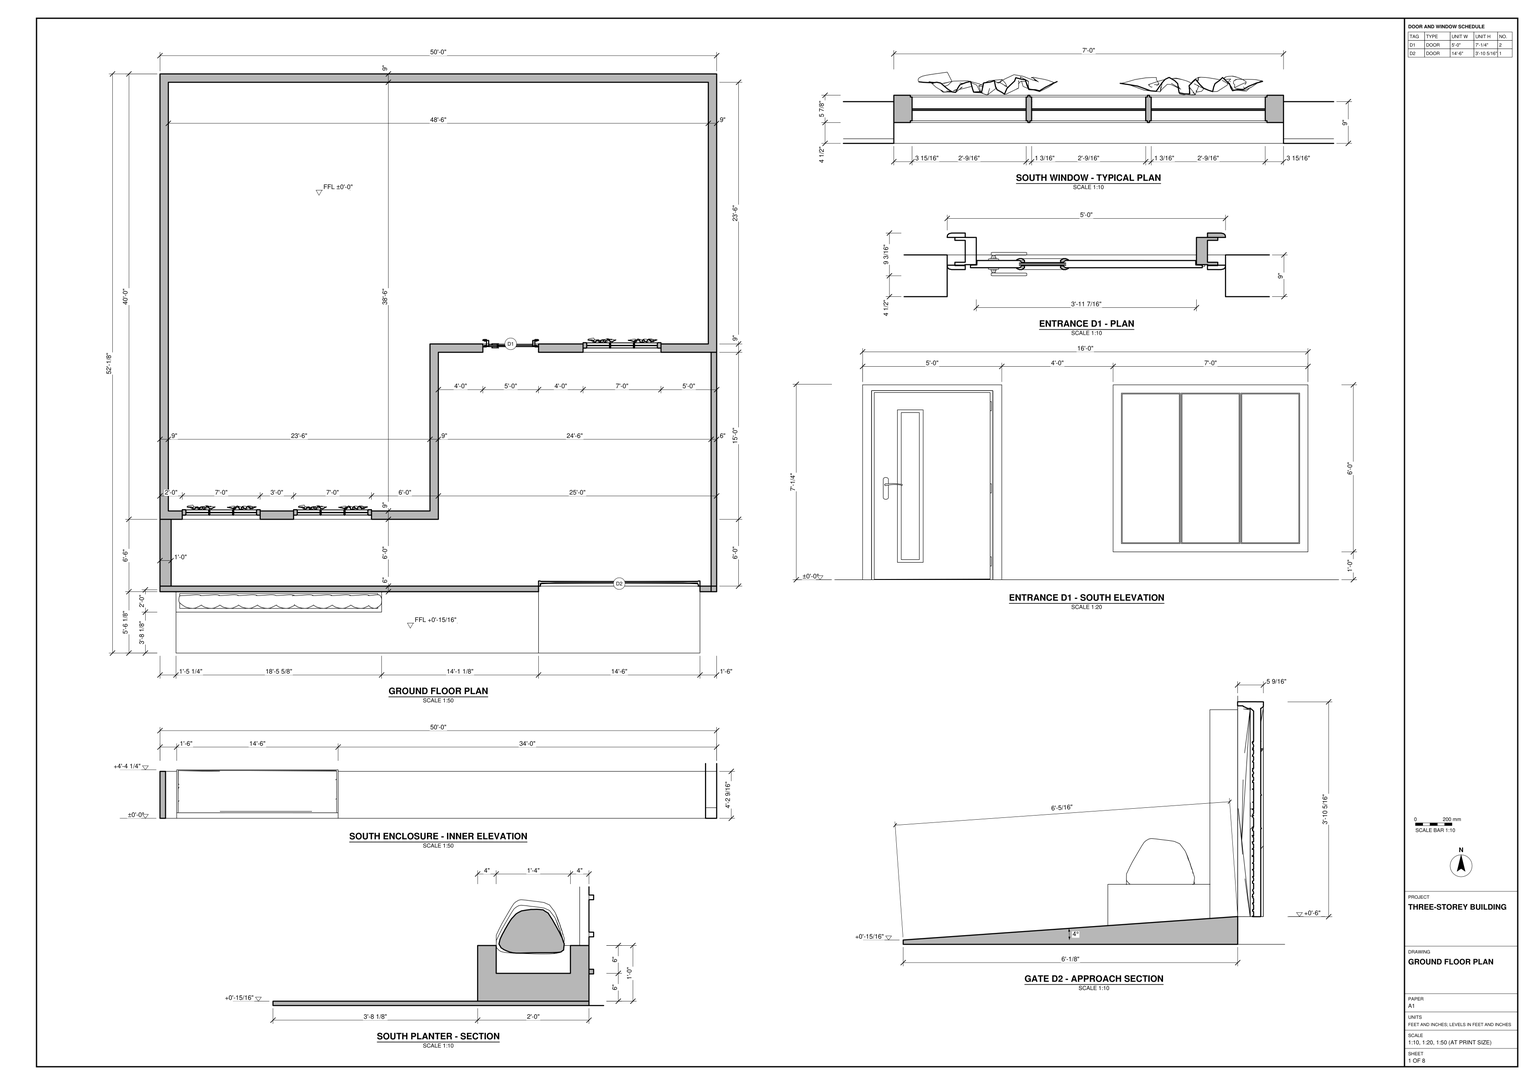
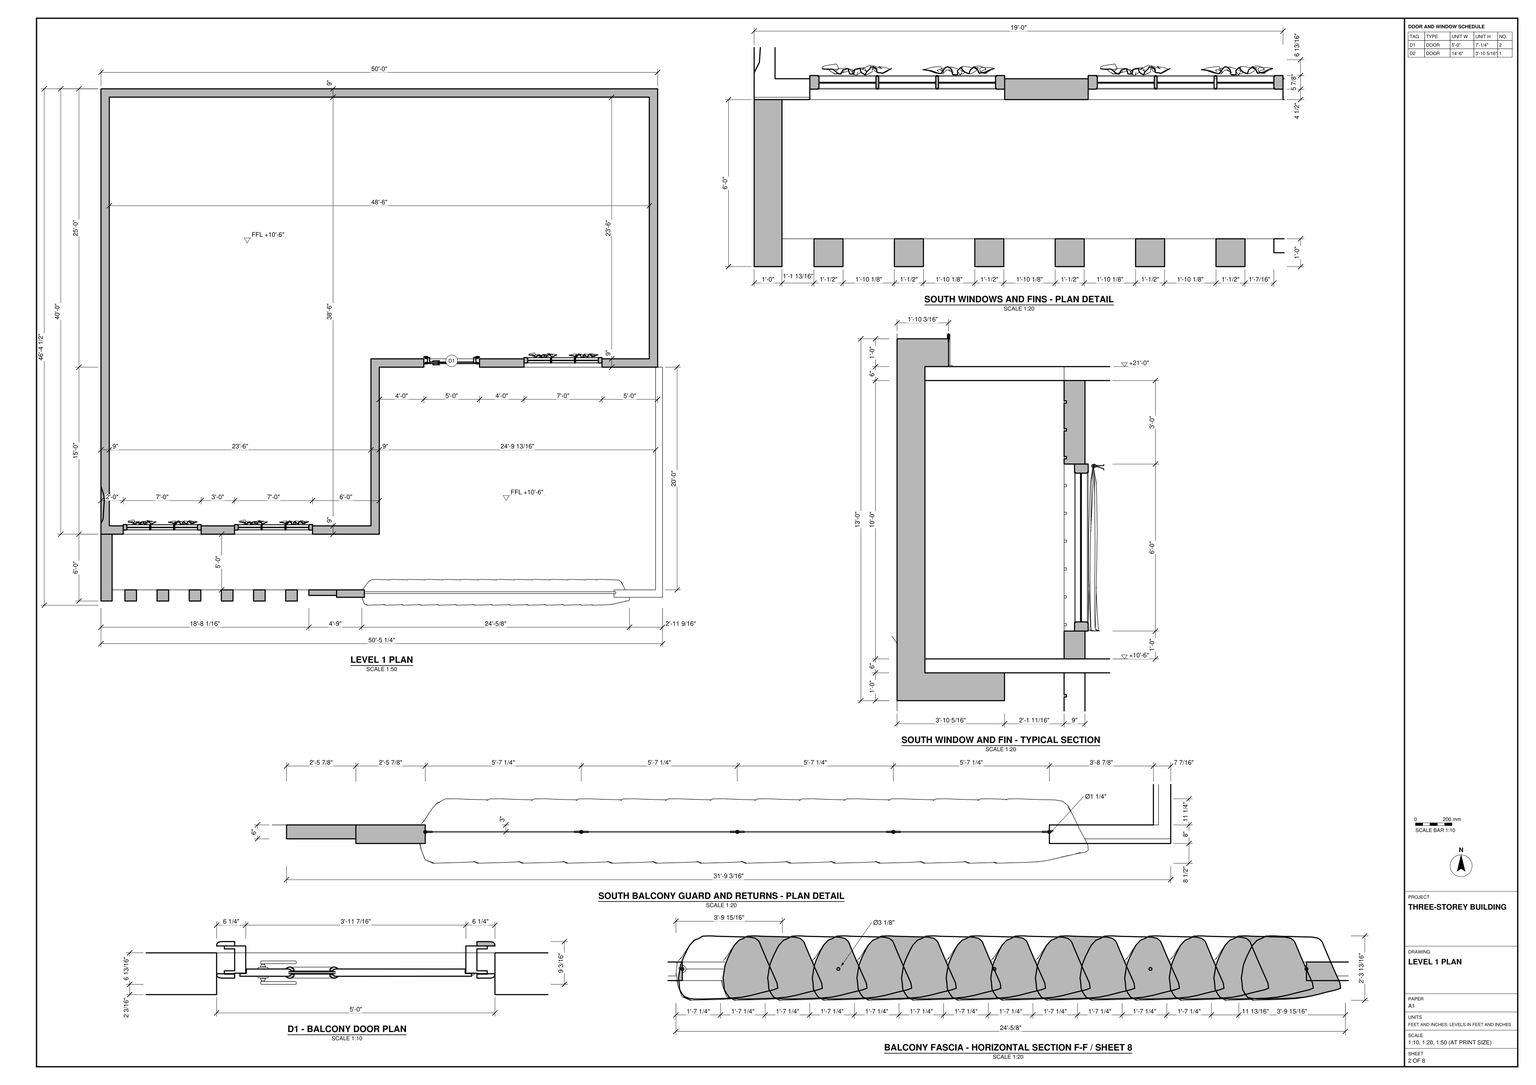
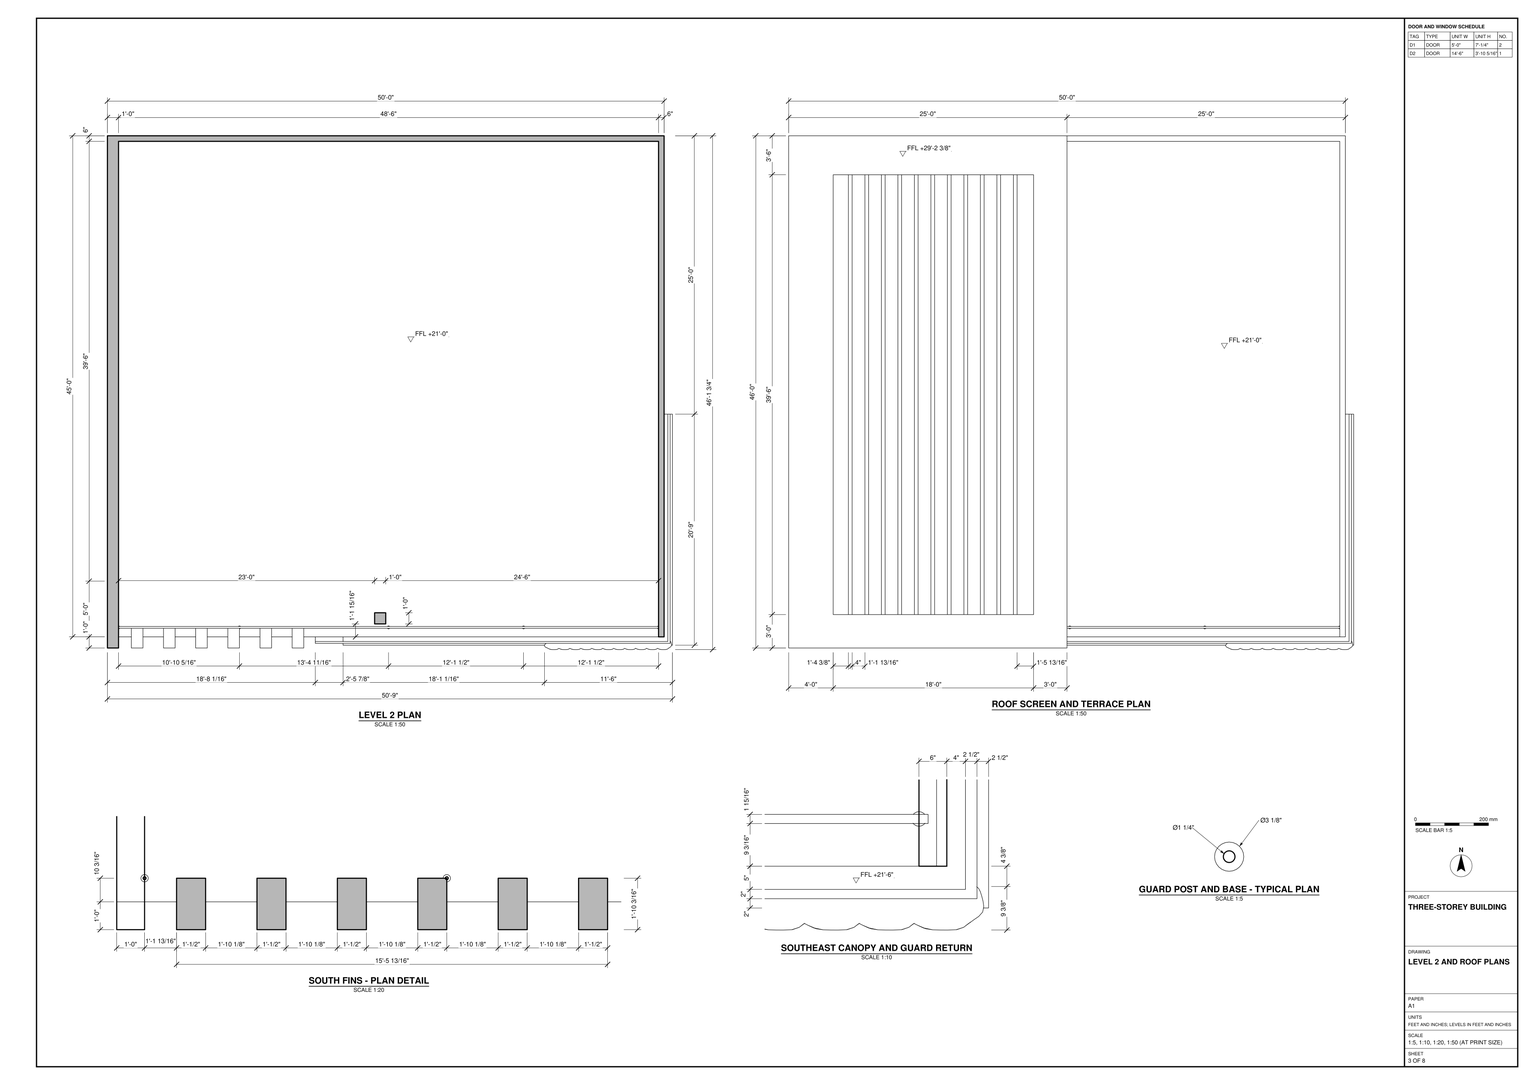
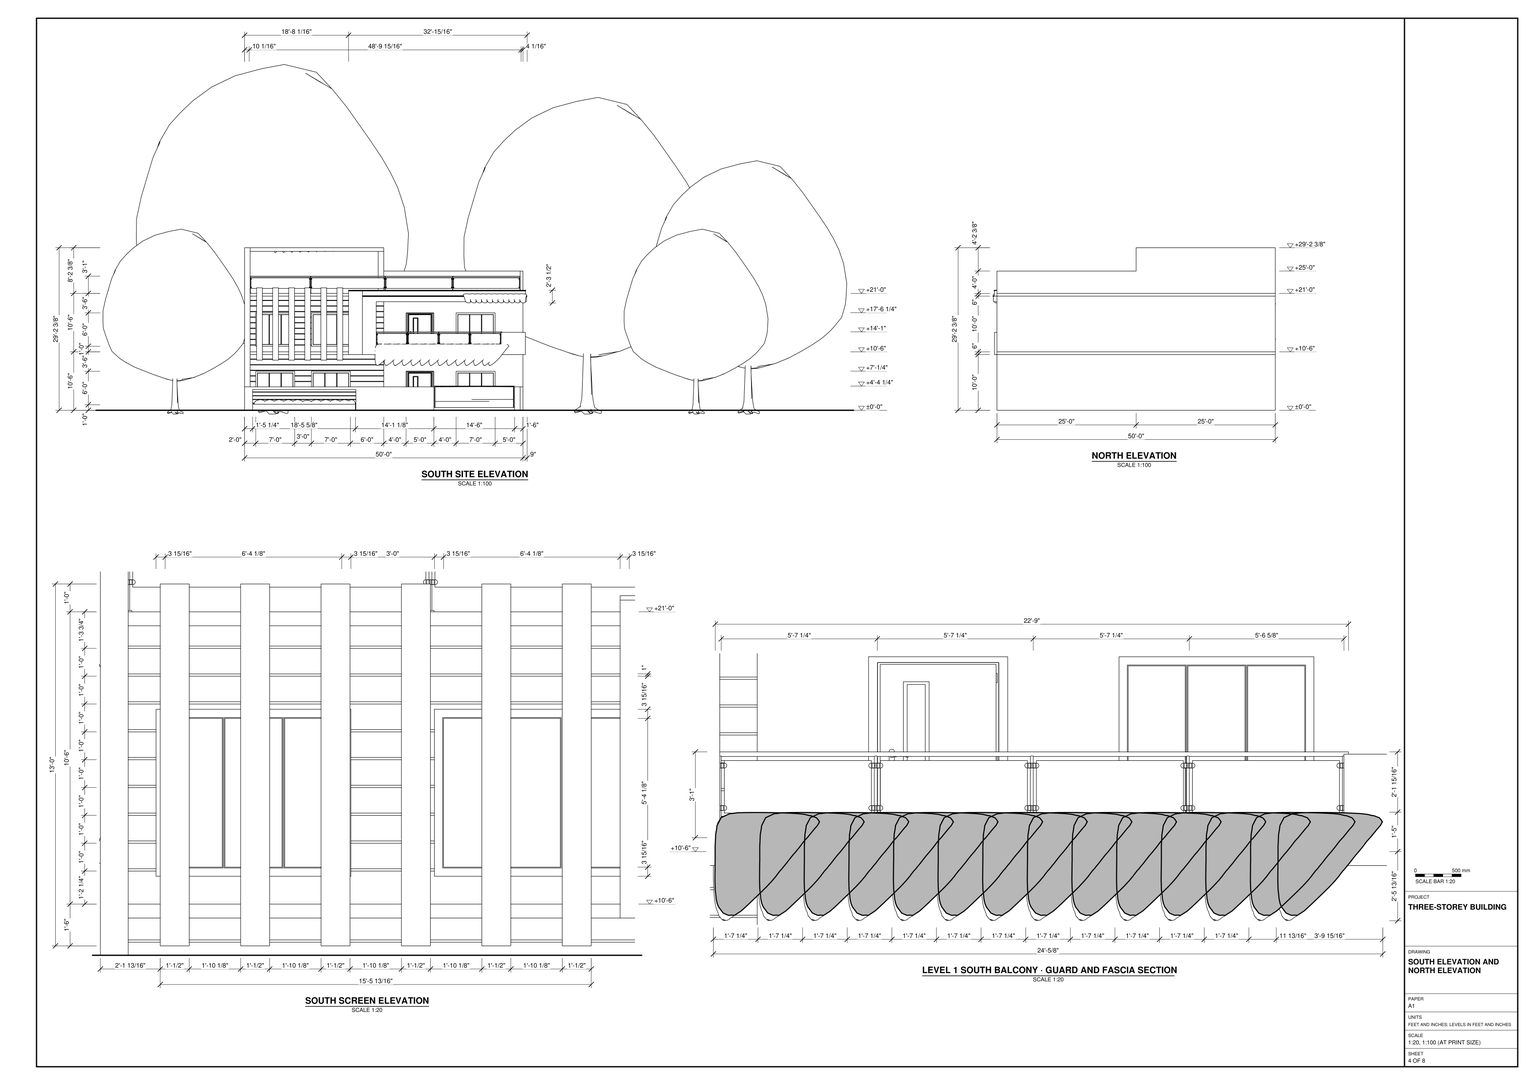
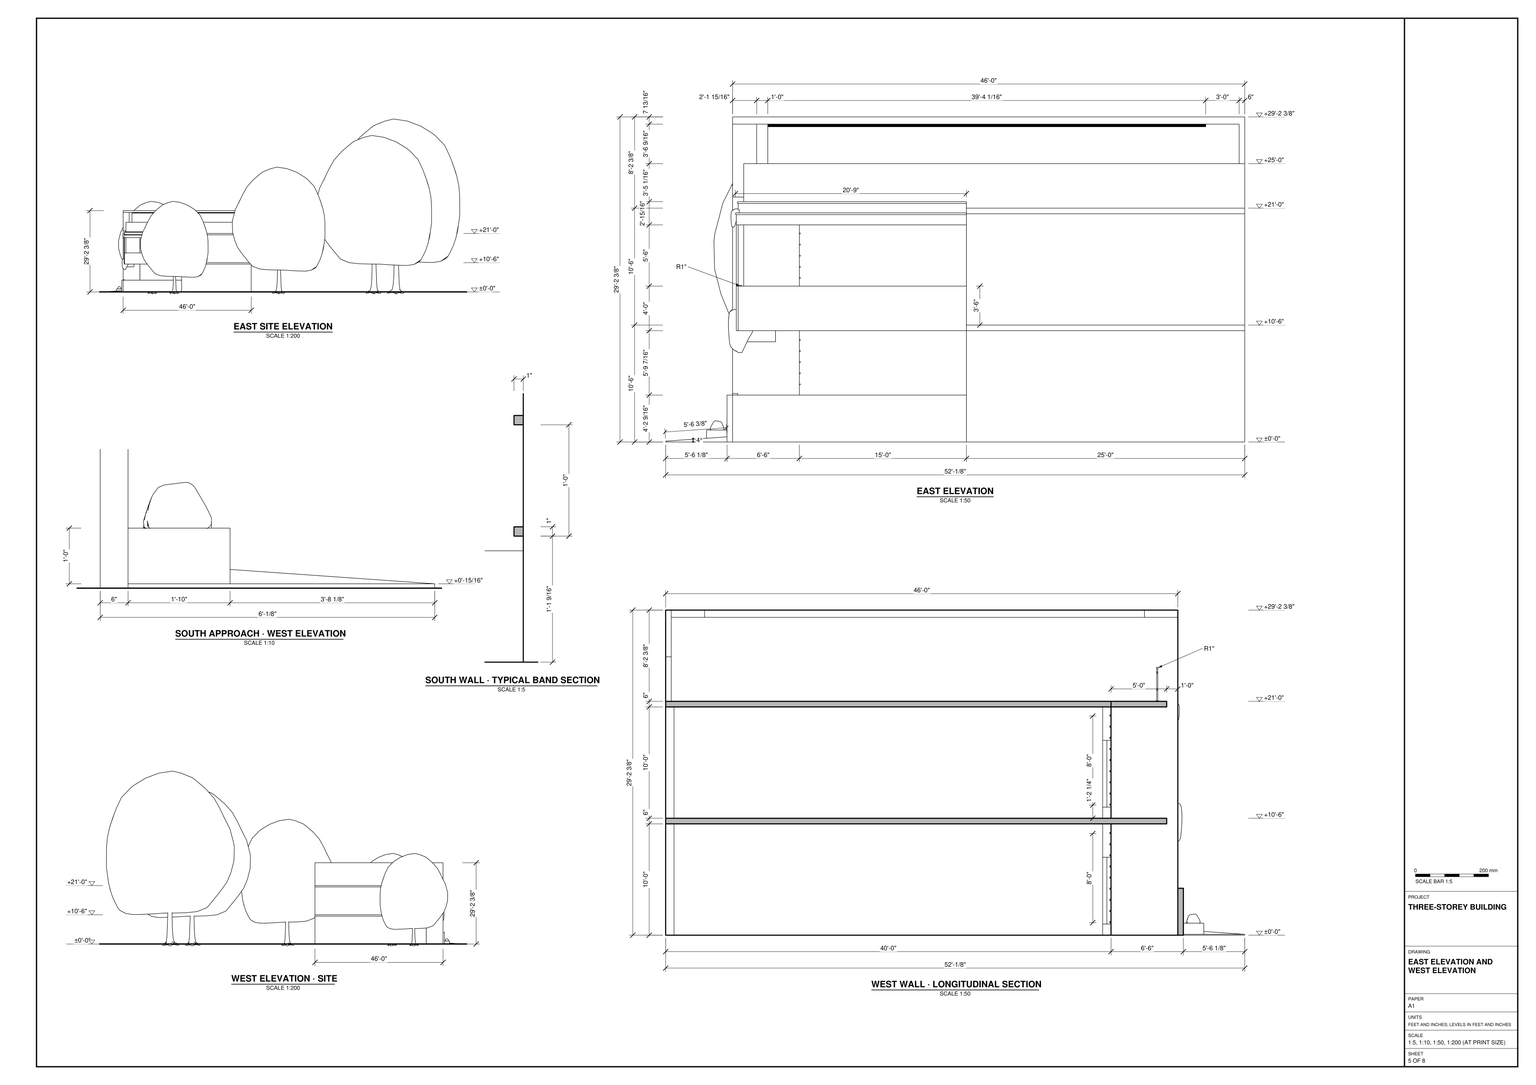
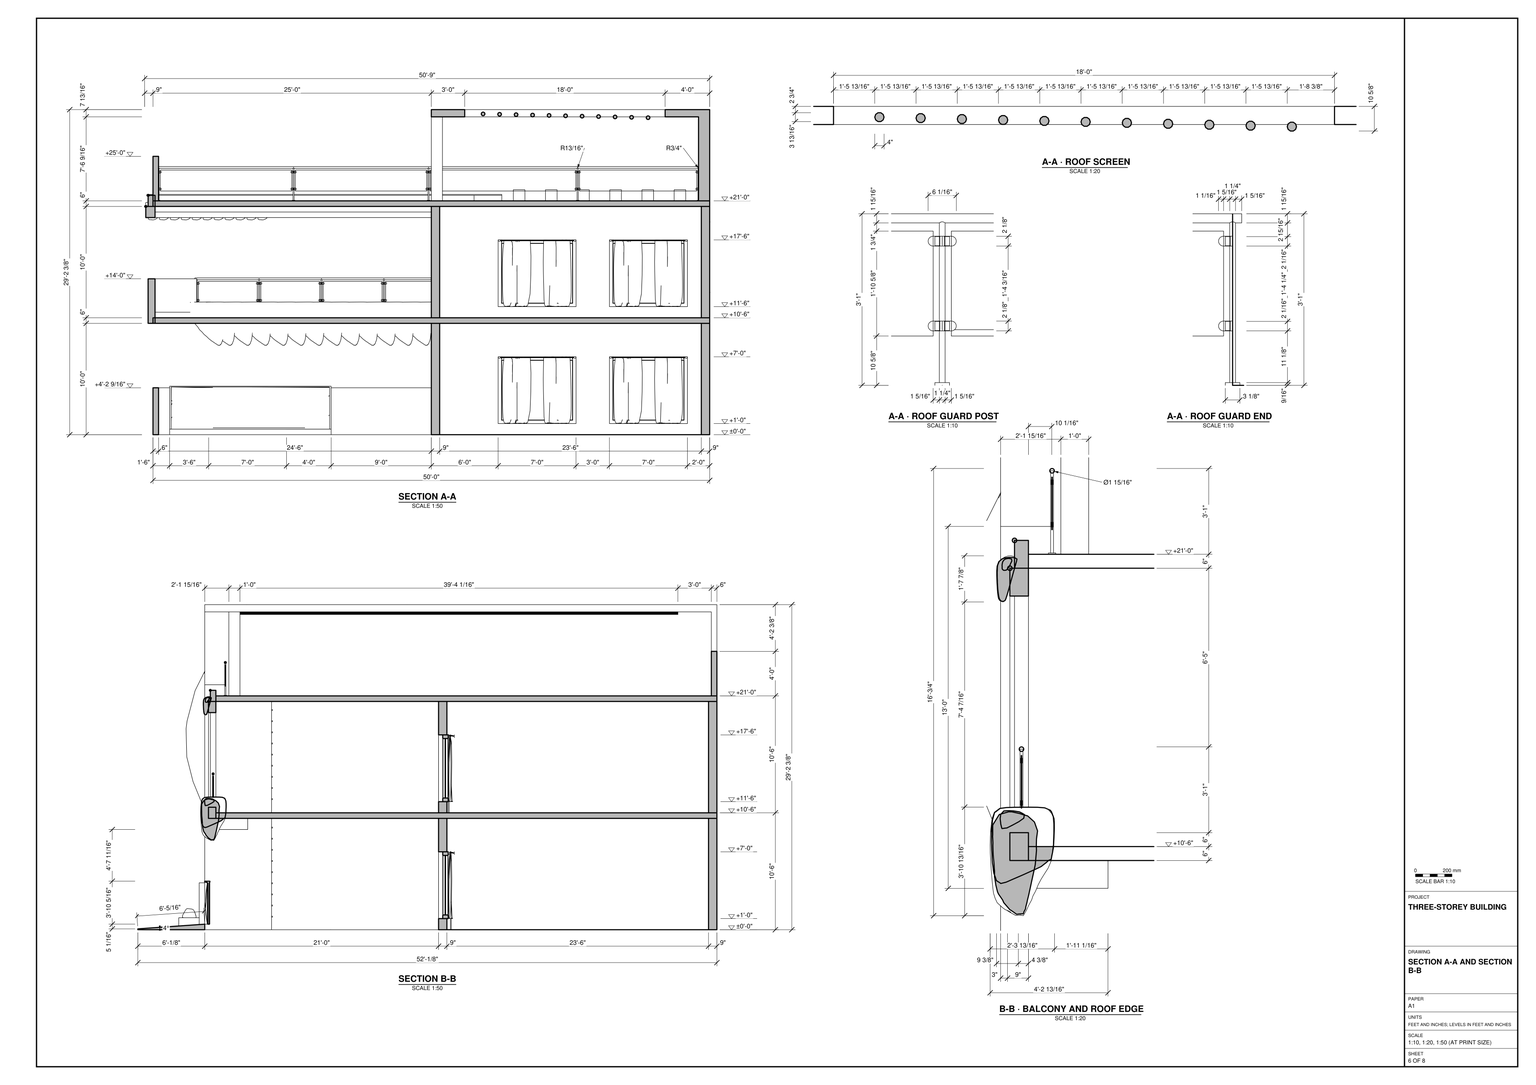
Build the three-storey building in SketchUp from task_files/diagram_01.pdf. Work in feet and inches. The complete model shall measure 133'-7 7/16" along X, 126'-11 1/8" along Y and 62'-9 9/16" along Z. These are the extents of the whole model, not the dimensions of the building footprint. Set the ground floor at ±0'-0", Level 1 at +10'-6" and Level 2 at +21'-0".

Use the floor plans to lay out the walls at their drawn thicknesses. On the two lower floors, the west wing projects south of the entrance wall. Fit the framed window units and doors into the wall openings. At ground level, model the south enclosure with the planter on the west and the sloping approach to the vehicle gate on the east.

Follow the sections for the floor slabs, projecting balcony edge and vertical fins in front of the Level 1 windows. Model the balcony's glass guard, its corner return and the repeating curved fascia. At roof level, distinguish the parallel strips of the roof screen on the west from the open terrace on the east. Decor and loose items, including planting and curtains, may be any suitable library components.

Keep shell elements such as walls, slabs and roof separate as groups or components. Keep each furniture or joinery piece shown separate, and use components for repeated parts. Save one SketchUp model as output_files/three_storey_building_south_balcony_and_roof_terrace.skp.

# SketchUp Ruby script. Lengths in inches.
U = 1.inch
M = Sketchup.active_model
def pt(a) = Geom::Point3d.new(a.map { |v| v * U })
def face(e, loops, mat)
  f = e.add_face(loops[0].map { |a| pt(a) })
  loops[1..].each { |l| e.add_face(l.map { |a| pt(a) }).erase! }
  f.material = f.back_material = mat if mat
  f
end
# faces: each face lists its corners as indices into pts; further lists are holes
def faces(e, pts, list, mat = nil) = list.each { |f| face(e, (f[0].is_a?(Array) ? f : [f]).map { |l| l.map { |i| pts[i] } }, mat) }
# xy, xz, yz: faces in a plane at the given z, y or x. An outline is a flat list of corners, or four numbers for a rectangle; further outlines are holes
def ring(l) = l.size == 4 ? [[l[0], l[1]], [l[2], l[1]], [l[2], l[3]], [l[0], l[3]]] : l.each_slice(2).to_a
def flat(e, list, mat, &to3) = list.each { |f| face(e, (f[0].is_a?(Array) ? f : [f]).map { |l| ring(l).map { |u, v| to3.(u, v) } }, mat) }
def xy(e, z, list, mat = nil) = flat(e, list, mat) { |x, y| [x, y, z] }
def xz(e, y, list, mat = nil) = flat(e, list, mat) { |x, z| [x, y, z] }
def yz(e, x, list, mat = nil) = flat(e, list, mat) { |y, z| [x, y, z] }
def lines(e, pts, list) = list.each { |a, b| e.add_line(pt(pts[a]), pt(pts[b])) }
# prism: a flat outline (further loops are holes) pulled along v
def prism(e, loops, v, mat = nil)
  f = face(e, loops, mat); d = Geom::Vector3d.new(v.map { |x| x * U })
  f.pushpull(f.normal.samedirection?(d) ? d.length : -d.length)
end
def box(e, o, s, mat = nil) = prism(e, [[o, [o[0] + s[0], o[1], o[2]], [o[0] + s[0], o[1] + s[1], o[2]], [o[0], o[1] + s[1], o[2]]]], [0, 0, s[2]], mat)
def at(x, y, z, deg = 0) = Geom::Transformation.translation(pt([x, y, z])) * Geom::Transformation.rotation(ORIGIN, Z_AXIS, deg.degrees)
def axes(o, x, y, z) = Geom::Transformation.new([*x, 0, *y, 0, *z, 0, *pt(o).to_a, 1])
def part(name) = M.definitions.add(name)
# library, detail: a bought-in or finely detailed component or shape, given as its bounding box
def library(name, o, s) = part(name).tap { |d| box(d.entities, o, s) }
def detail(e, o, s) = box(e.add_group.entities, o, s)
def put(e, d, t, mat = nil) = e.add_instance(d, t).tap { |i| i.material = mat if mat }
def group(e, t, mat = nil) = e.add_group.tap { |g| g.transformation = t; g.material = mat if mat }.entities
root = M.entities
M.materials.add("Marble White 604 35.18cm").color = [255, 255, 255]
M.materials.add("Metal for window").color = [30, 30, 30]
M.materials.add("Wall Paint Dusk Blue Matte 300cm").color = [122, 143, 157]
M.materials.add("Wall Paint Fine Grain 01 White 100cm").color = [188, 188, 188]
M.materials.add("Wall Paint Fine Grain 01 Yellow 100cm").color = [207, 190, 139]
c1 = library("Window with curtains",[-42,-36,-6.8],[84,72,12.68])
c2 = part("Component\#3")
prism(c2.entities,[[[0,-12,144],[0,10.1875,144],[0,10.1875,132],[0,0,132],[0,0,0],[0,34.3125,0],[0,34.3125,-12],[0,-12,-12]]],[12.51,0,0],"Wall Paint Dusk Blue Matte 300cm")
c3 = library("Door 29",[-21.26,-5.27,0],[42.52,9.21,84.25])
c4 = library("Lithodora diffusa 002",[-13.17,-15.15,-0.88],[26.36,28.16,10.5])
c5 = library("Viola hederacea 012",[-7.68,-13.51,-41.79],[45.92,27.79,46.82])
c6 = library("Dichondra repens 010",[-9.09,-7.76,-17.89],[18.82,9.4,19.89])
c7 = library("Garage Gate 243 109",[-100.16,-2.78,0],[200.32,5.56,100.68])
c8 = library("Tilia x europaea Pallida 002",[-155.08,-146.63,-8.22],[310.29,291.58,398.59])
c9 = part("Group13\#2")
prism(c9.entities,[[[111.79,-6.08,346.72],[111.4,-6.08,345.54],[111.79,-6.08,344.36],[112.79,-6.08,343.64],[114.02,-6.08,343.64],[115.02,-6.08,344.36],[115.4,-6.08,345.54],[115.02,-6.08,346.72],[114.02,-6.08,347.44],[112.79,-6.08,347.44]]],[0,474,0])
c10 = part("Group13\#1")
prism(c10.entities,[[[111.79,-6.08,346.72],[111.4,-6.08,345.54],[111.79,-6.08,344.36],[112.79,-6.08,343.64],[114.02,-6.08,343.64],[115.02,-6.08,344.36],[115.4,-6.08,345.54],[115.02,-6.08,346.72],[114.02,-6.08,347.44],[112.79,-6.08,347.44]]],[0,474,0])
c11 = part("Group10\#1")
xy(c11.entities,245.05,[[353.4,-38.39,353.4,-37.77,637.09,-37.77,637.09,209.92,637.71,209.92,637.71,-38.39]])
xy(c11.entities,246.95,[[353.4,-38.39,637.71,-38.39,637.71,209.92,637.09,209.92,637.09,-37.77,353.4,-37.77]])
xz(c11.entities,209.92,[[637.09,245.05,636.59,245.41,636.4,246,636.59,246.59,637.09,246.95,637.71,246.95,638.21,246.59,638.4,246,638.21,245.41,637.71,245.05]])
yz(c11.entities,353.4,[[-38.39,245.05,-38.89,245.41,-39.08,246,-38.89,246.59,-38.39,246.95,-37.77,246.95,-37.27,246.59,-37.08,246,-37.27,245.41,-37.77,245.05]])
p = [[637.71,-38.39,245.05],[638.21,-38.89,245.41],[353.4,-38.89,245.41],[353.4,-38.39,245.05],[637.71,209.92,245.05],[638.21,209.92,245.41],
  [636.59,-37.27,245.41],[637.09,-37.77,245.05],[353.4,-37.77,245.05],[353.4,-37.27,245.41],[636.59,209.92,245.41],[637.09,209.92,245.05],
  [638.4,-39.08,246],[353.4,-39.08,246],[638.4,209.92,246],[636.4,-37.08,246],[353.4,-37.08,246],[636.4,209.92,246],
  [638.21,-38.89,246.59],[353.4,-38.89,246.59],[638.21,209.92,246.59],[636.59,-37.27,246.59],[353.4,-37.27,246.59],[636.59,209.92,246.59],
  [637.71,-38.39,246.95],[353.4,-38.39,246.95],[637.71,209.92,246.95],[637.09,-37.77,246.95],[353.4,-37.77,246.95],[637.09,209.92,246.95]]
faces(c11.entities,p,[[0,1,2,3],[4,5,1,0],[6,7,8,9],[10,11,7,6],[1,12,13,2],[5,14,12,1],[15,6,9,16],[17,10,6,15],
  [12,18,19,13],[14,20,18,12],[21,15,16,22],[23,17,15,21],[18,24,25,19],[20,26,24,18],[27,21,22,28],[29,23,21,27]])
c12 = part("Group11\#1")
xy(c12.entities,257.05,[[329.4,-36.39,329.4,-35.77,635.09,-35.77,635.09,209.92,635.71,209.92,635.71,-36.39]])
xy(c12.entities,258.95,[[329.4,-36.39,635.71,-36.39,635.71,209.92,635.09,209.92,635.09,-35.77,329.4,-35.77]])
xz(c12.entities,209.92,[[635.09,257.05,634.59,257.41,634.4,258,634.59,258.59,635.09,258.95,635.71,258.95,636.21,258.59,636.4,258,636.21,257.41,635.71,257.05]])
yz(c12.entities,329.4,[[-36.39,257.05,-36.89,257.41,-37.08,258,-36.89,258.59,-36.39,258.95,-35.77,258.95,-35.27,258.59,-35.08,258,-35.27,257.41,-35.77,257.05]])
p = [[329.4,-36.89,257.41],[329.4,-36.39,257.05],[353.4,-36.39,257.05],[635.71,-36.39,257.05],[636.21,-36.89,257.41],[353.4,-36.89,257.41],
  [635.71,209.92,257.05],[636.21,209.92,257.41],[329.4,-35.77,257.05],[329.4,-35.27,257.41],[353.4,-35.27,257.41],[634.59,-35.27,257.41],
  [635.09,-35.77,257.05],[353.4,-35.77,257.05],[634.59,209.92,257.41],[635.09,209.92,257.05],[329.4,-37.08,258],[636.4,-37.08,258],
  [353.4,-37.08,258],[636.4,209.92,258],[353.4,-35.08,258],[634.4,-35.08,258],[329.4,-35.08,258],[634.4,209.92,258],
  [329.4,-36.89,258.59],[636.21,-36.89,258.59],[353.4,-36.89,258.59],[636.21,209.92,258.59],[353.4,-35.27,258.59],[634.59,-35.27,258.59],
  [329.4,-35.27,258.59],[634.59,209.92,258.59],[329.4,-36.39,258.95],[635.71,-36.39,258.95],[353.4,-36.39,258.95],[635.71,209.92,258.95],
  [353.4,-35.77,258.95],[635.09,-35.77,258.95],[329.4,-35.77,258.95],[635.09,209.92,258.95]]
faces(c12.entities,p,[[0,1,2,3,4,5],[4,3,6,7],[8,9,10,11,12,13],[12,11,14,15],[16,0,5,4,17,18],[17,4,7,19],[20,21,11,10,9,22],[11,21,23,14],
  [24,16,18,17,25,26],[25,17,19,27],[28,29,21,20,22,30],[21,29,31,23],[32,24,26,25,33,34],[33,25,27,35],[36,37,29,28,30,38],[29,37,39,31]])
c13 = library("Group\#11",[0,0,0],[273.02,3.15,36.98])
c14 = library("Group\#12",[0,0,0],[585.9375,3.15,36.98])
p = [[24,144.12,12],[24,144.12,84],[108,144.12,84],[108,144.12,12],[348,324.12,0],[348,324.12,84],
  [408,324.12,84],[408,324.12,0],[12,79.13,0],[12,78.12,0]]
lines(root,p,[[0,1],[1,2],[2,3],[3,0],[4,5],[5,6],[6,7],[7,4],[8,9]])
put(root,c1,axes([66,154.49,48],[1,0,0],[0,0,1],[0,-1,0]))
put(root,c1,axes([186,154.49,48],[1,0,0],[0,0,1],[0,-1,0]))
put(root,c1,axes([498,334.49,48],[1,0,0],[0,0,1],[0,-1,0]))
put(root,c1,axes([498,334.49,174],[1,0,0],[0,0,1],[0,-1,0]))
put(root,c1,axes([66,154.49,174],[1,0,0],[0,0,1],[0,-1,0]))
put(root,c1,axes([186,154.49,174],[1,0,0],[0,0,1],[0,-1,0]))
put(root,c2,at(25.8,84.12,120))
put(root,c2,at(60.46,84.12,120))
put(root,c2,at(95.12,84.12,120))
put(root,c2,at(129.78,84.12,120))
put(root,c2,at(164.45,84.12,120))
put(root,c2,at(199.11,84.12,120))
put(root,c3,axes([378,333.89,0],[1.41111,0,0],[0,1,0],[0,0,1]))
put(root,c3,axes([378,331.61,126],[1.41111,0,0],[0,1,0],[0,0,1]))
put(root,c4,axes([33.46,56.02,13.1875],[1,0,0],[0,0.52197,0],[0,0,1]))
put(root,c4,axes([53.625,56.02,13.1875],[1,0,0],[0,0.52197,0],[0,0,1]))
put(root,c4,axes([73.79,56.02,13.1875],[1,0,0],[0,0.52197,0],[0,0,1]))
put(root,c4,axes([93.95,56.02,13.1875],[1,0,0],[0,0.52197,0],[0,0,1]))
put(root,c4,axes([114.12,56.02,13.1875],[1,0,0],[0,0.52197,0],[0,0,1]))
put(root,c4,axes([134.28,56.02,12],[1,0,0],[0,0.52197,0],[0,0,1]))
put(root,c4,axes([154.45,56.02,13.1875],[1,0,0],[0,0.52197,0],[0,0,1]))
put(root,c4,axes([174.61,56.02,13.1875],[1,0,0],[0,0.52197,0],[0,0,1]))
put(root,c4,axes([194.78,56.02,13.1875],[1,0,0],[0,0.52197,0],[0,0,1]))
put(root,c4,axes([214.9375,56.02,13.1875],[1,0,0],[0,0.52197,0],[0,0,1]))
put(root,c4,axes([230.4,56.02,13.1875],[0.64265,0,0],[0,0.52197,0],[0,0,1]))
put(root,c5,at(288.77,81.12,138))
put(root,c5,at(308.01,81.12,138))
put(root,c5,at(327.25,81.12,138))
put(root,c5,at(346.49,81.12,138))
put(root,c5,at(365.73,81.12,138))
put(root,c5,at(384.96,81.12,138))
put(root,c5,at(404.2,81.12,138))
put(root,c5,at(423.44,81.12,138))
put(root,c5,at(442.68,81.12,138))
put(root,c5,at(461.92,81.12,138))
put(root,c5,at(481.16,81.12,138))
put(root,c5,at(500.39,81.12,138))
put(root,c5,at(519.63,81.12,138))
put(root,c5,at(531.45,81.12,138))
put(root,c6,at(598.24,78.12,249.36))
put(root,c6,at(586.42,78.12,249.36))
put(root,c6,at(574.61,78.12,249.36))
put(root,c6,at(562.8,78.12,249.36))
put(root,c6,at(550.99,78.12,249.36))
put(root,c6,at(539.17,78.12,249.36))
put(root,c6,at(527.36,78.12,249.36))
put(root,c6,at(515.55,78.12,249.36))
put(root,c6,at(503.74,78.12,249.36))
put(root,c6,at(491.92,78.12,249.36))
put(root,c6,at(480.11,78.12,249.36))
put(root,c7,axes([495,74.87,5.97],[0.86859,0,0],[0,1,0],[0,0,0.46]))
put(root,c8,at(-150.27,198.61,0))
put(root,c8,axes([59.88,1249.11,7.32],[1.8906,0,0],[0,1.8906,0],[0,0,1.8906]))
put(root,c8,axes([738.25,1153.49,5.85],[1.7125,0,0],[0,1.7125,0],[0,0,1.7125]))
put(root,c8,axes([1085.46,743.65,3.04],[1.37,0,0],[0,1.37,0],[0,0,1.37]))
put(root,c8,at(973.15,293.29,0))
g1 = group(root,at(0,144.12,0))
xy(g1,0,[[0,0,0,480,600,480,600,180,408,180,408,189,591,189,591,471,9,471,9,9,291,9,291,189,348,189,348,180,300,180,300,0],[9,9,291,9,291,189,591,189,591,471,9,471]])
xy(g1,12,[[456,180,540,189]])
xy(g1,12,[[24,0,108,9],[144,0,228,9]],"Wall Paint Fine Grain 01 Yellow 100cm")
xy(g1,13.58,[[0,0,24,1],[108,0,144,1],[228,0,300,1]],"Wall Paint Fine Grain 01 Yellow 100cm")
xy(g1,14.58,[[0,0,24,1],[108,0,144,1],[228,0,300,1]],"Wall Paint Fine Grain 01 Yellow 100cm")
xy(g1,25.58,[[0,0,24,1],[108,0,144,1],[228,0,300,1]],"Wall Paint Fine Grain 01 Yellow 100cm")
xy(g1,26.58,[[0,0,24,1],[108,0,144,1],[228,0,300,1]],"Wall Paint Fine Grain 01 Yellow 100cm")
xy(g1,37.58,[[0,0,24,1],[108,0,144,1],[228,0,300,1]],"Wall Paint Fine Grain 01 Yellow 100cm")
xy(g1,38.58,[[0,0,24,1],[108,0,144,1],[228,0,300,1]],"Wall Paint Fine Grain 01 Yellow 100cm")
xy(g1,49.58,[[0,0,24,1],[108,0,144,1],[228,0,300,1]],"Wall Paint Fine Grain 01 Yellow 100cm")
xy(g1,50.58,[[0,0,24,1],[108,0,144,1],[228,0,300,1]],"Wall Paint Fine Grain 01 Yellow 100cm")
xy(g1,61.58,[[0,0,24,1],[108,0,144,1],[228,0,300,1]],"Wall Paint Fine Grain 01 Yellow 100cm")
xy(g1,62.58,[[0,0,24,1],[108,0,144,1],[228,0,300,1]],"Wall Paint Fine Grain 01 Yellow 100cm")
xy(g1,73.58,[[0,0,24,1],[108,0,144,1],[228,0,300,1]],"Wall Paint Fine Grain 01 Yellow 100cm")
xy(g1,74.58,[[0,0,24,1],[108,0,144,1],[228,0,300,1]],"Wall Paint Fine Grain 01 Yellow 100cm")
xy(g1,84,[[348,180,408,189],[456,180,540,189]])
xy(g1,84,[[24,0,108,9],[144,0,228,9]],"Wall Paint Fine Grain 01 Yellow 100cm")
xy(g1,85.58,[[0,0,300,1]],"Wall Paint Fine Grain 01 Yellow 100cm")
xy(g1,86.58,[[0,0,300,1]],"Wall Paint Fine Grain 01 Yellow 100cm")
xy(g1,97.58,[[0,0,300,1]],"Wall Paint Fine Grain 01 Yellow 100cm")
xy(g1,98.58,[[0,0,300,1]],"Wall Paint Fine Grain 01 Yellow 100cm")
xy(g1,109.58,[[0,0,300,1]],"Wall Paint Fine Grain 01 Yellow 100cm")
xy(g1,110.58,[[0,0,300,1]],"Wall Paint Fine Grain 01 Yellow 100cm")
xy(g1,120,[[[0,0,300,0,300,180,600,180,600,480,0,480],[9,9,9,471,591,471,591,189,291,189,291,9]]])
xz(g1,0,[[0,0,300,0,300,13.58,228,13.58,228,12,144,12,144,13.58,108,13.58,108,12,24,12,24,13.58,0,13.58],[0,14.58,24,25.58],[108,14.58,144,25.58],[228,14.58,300,25.58],[0,26.58,24,37.58],
  [108,26.58,144,37.58],[228,26.58,300,37.58],[0,38.58,24,49.58],[108,38.58,144,49.58],[228,38.58,300,49.58],
  [0,50.58,24,61.58],[108,50.58,144,61.58],[228,50.58,300,61.58],[0,62.58,24,73.58],[108,62.58,144,73.58],
  [228,62.58,300,73.58],[0,74.58,24,74.58,24,84,108,84,108,74.58,144,74.58,144,84,228,84,228,74.58,300,74.58,300,85.58,0,85.58],[0,86.58,300,97.58],[0,98.58,300,109.58],[0,110.58,300,120]],"Wall Paint Fine Grain 01 Yellow 100cm")
xz(g1,1,[[0,13.58,24,14.58],[108,13.58,144,14.58],[228,13.58,300,14.58],[0,25.58,24,26.58],[108,25.58,144,26.58],
  [228,25.58,300,26.58],[0,37.58,24,38.58],[108,37.58,144,38.58],[228,37.58,300,38.58],[0,49.58,24,50.58],
  [108,49.58,144,50.58],[228,49.58,300,50.58],[0,61.58,24,62.58],[108,61.58,144,62.58],[228,61.58,300,62.58],
  [0,73.58,24,74.58],[108,73.58,144,74.58],[228,73.58,300,74.58],[0,85.58,300,86.58],[0,97.58,300,98.58],
  [0,109.58,300,110.58]],"Wall Paint Fine Grain 01 Yellow 100cm")
xz(g1,9,[[[9,0,291,120],[24,12,108,84],[144,12,228,84]]],"Wall Paint Fine Grain 01 Yellow 100cm")
xz(g1,180,[[[300,0,348,0,348,84,408,84,408,0,600,0,600,120,300,120],[456,12,540,84]]],"Wall Paint Fine Grain 01 White 100cm")
xz(g1,189,[[[291,0,291,120,591,120,591,0,408,0,408,84,348,84,348,0],[456,12,540,84]]])
xz(g1,471,[[9,0,591,120]])
xz(g1,480,[[0,0,600,120]])
yz(g1,0,[[0,0,0,13.58,1,13.58,1,14.58,0,14.58,0,25.58,1,25.58,1,26.58,0,26.58,0,37.58,1,37.58,1,38.58,0,38.58,0,49.58,1,49.58,1,50.58,0,50.58,0,61.58,1,61.58,1,62.58,0,62.58,0,73.58,1,73.58,1,74.58,0,74.58,0,85.58,1,85.58,1,86.58,0,86.58,0,97.58,1,97.58,1,98.58,0,98.58,0,109.58,1,109.58,1,110.58,0,110.58,0,120,480,120,480,0]])
yz(g1,0,[[0,13.58,1,14.58],[0,25.58,1,26.58],[0,37.58,1,38.58],[0,49.58,1,50.58],[0,61.58,1,62.58],
  [0,73.58,1,74.58],[0,85.58,1,86.58],[0,97.58,1,98.58],[0,109.58,1,110.58]],"Wall Paint Fine Grain 01 Yellow 100cm")
yz(g1,9,[[9,0,471,120]])
yz(g1,24,[[0,12,9,12,9,84,0,84,0,74.58,1,74.58,1,73.58,0,73.58,0,62.58,1,62.58,1,61.58,0,61.58,0,50.58,1,50.58,1,49.58,0,49.58,0,38.58,1,38.58,1,37.58,0,37.58,0,26.58,1,26.58,1,25.58,0,25.58,0,14.58,1,14.58,1,13.58,0,13.58],[0,13.58,1,14.58],[0,25.58,1,26.58],[0,37.58,1,38.58],[0,49.58,1,50.58],
  [0,61.58,1,62.58],[0,73.58,1,74.58]],"Wall Paint Fine Grain 01 Yellow 100cm")
yz(g1,108,[[0,12,0,13.58,1,13.58,1,14.58,0,14.58,0,25.58,1,25.58,1,26.58,0,26.58,0,37.58,1,37.58,1,38.58,0,38.58,0,49.58,1,49.58,1,50.58,0,50.58,0,61.58,1,61.58,1,62.58,0,62.58,0,73.58,1,73.58,1,74.58,0,74.58,0,84,9,84,9,12],[0,13.58,1,14.58],[0,25.58,1,26.58],[0,37.58,1,38.58],[0,49.58,1,50.58],
  [0,61.58,1,62.58],[0,73.58,1,74.58]],"Wall Paint Fine Grain 01 Yellow 100cm")
yz(g1,144,[[0,12,9,12,9,84,0,84,0,74.58,1,74.58,1,73.58,0,73.58,0,62.58,1,62.58,1,61.58,0,61.58,0,50.58,1,50.58,1,49.58,0,49.58,0,38.58,1,38.58,1,37.58,0,37.58,0,26.58,1,26.58,1,25.58,0,25.58,0,14.58,1,14.58,1,13.58,0,13.58],[0,13.58,1,14.58],[0,25.58,1,26.58],[0,37.58,1,38.58],[0,49.58,1,50.58],
  [0,61.58,1,62.58],[0,73.58,1,74.58]],"Wall Paint Fine Grain 01 Yellow 100cm")
yz(g1,228,[[0,12,0,13.58,1,13.58,1,14.58,0,14.58,0,25.58,1,25.58,1,26.58,0,26.58,0,37.58,1,37.58,1,38.58,0,38.58,0,49.58,1,49.58,1,50.58,0,50.58,0,61.58,1,61.58,1,62.58,0,62.58,0,73.58,1,73.58,1,74.58,0,74.58,0,84,9,84,9,12],[0,13.58,1,14.58],[0,25.58,1,26.58],[0,37.58,1,38.58],[0,49.58,1,50.58],
  [0,61.58,1,62.58],[0,73.58,1,74.58]],"Wall Paint Fine Grain 01 Yellow 100cm")
yz(g1,291,[[9,0,189,120]])
yz(g1,300,[[0,0,180,0,180,120,0,120,0,110.58,1,110.58,1,109.58,0,109.58,0,98.58,1,98.58,1,97.58,0,97.58,0,86.58,1,86.58,1,85.58,0,85.58,0,74.58,1,74.58,1,73.58,0,73.58,0,62.58,1,62.58,1,61.58,0,61.58,0,50.58,1,50.58,1,49.58,0,49.58,0,38.58,1,38.58,1,37.58,0,37.58,0,26.58,1,26.58,1,25.58,0,25.58,0,14.58,1,14.58,1,13.58,0,13.58],[0,13.58,1,14.58],[0,25.58,1,26.58],[0,37.58,1,38.58],[0,49.58,1,50.58],
  [0,61.58,1,62.58],[0,73.58,1,74.58],[0,85.58,1,86.58],[0,97.58,1,98.58],[0,109.58,1,110.58]],"Wall Paint Fine Grain 01 Yellow 100cm")
yz(g1,348,[[180,0,189,84]])
yz(g1,408,[[180,0,189,84]])
yz(g1,456,[[180,12,189,84]])
yz(g1,540,[[180,12,189,84]])
yz(g1,591,[[189,0,471,120]])
yz(g1,600,[[180,0,480,120]],"Wall Paint Fine Grain 01 White 100cm")
g2 = group(root,at(0,144.12,120))
box(g2,[0,-60,0],[600,540,6])
g3 = group(root,at(0,144.12,126))
xy(g3,0,[[0,0,0,480,600,480,600,180,408,180,408,189,591,189,591,471,9,471,9,9,291,9,291,189,348,189,348,180,300,180,300,0],[9,9,291,9,291,189,591,189,591,471,9,471]])
xy(g3,12,[[456,180,540,189]])
xy(g3,12,[[24,0,108,9],[144,0,228,9]],"Wall Paint Fine Grain 01 Yellow 100cm")
xy(g3,14.24,[[0,0,24,1],[108,0,144,1],[228,0,300,1]],"Wall Paint Fine Grain 01 Yellow 100cm")
xy(g3,15.24,[[0,0,24,1],[108,0,144,1],[228,0,300,1]],"Wall Paint Fine Grain 01 Yellow 100cm")
xy(g3,26.24,[[0,0,24,1],[108,0,144,1],[228,0,300,1]],"Wall Paint Fine Grain 01 Yellow 100cm")
xy(g3,27.24,[[0,0,24,1],[108,0,144,1],[228,0,300,1]],"Wall Paint Fine Grain 01 Yellow 100cm")
xy(g3,38.24,[[0,0,24,1],[108,0,144,1],[228,0,300,1]],"Wall Paint Fine Grain 01 Yellow 100cm")
xy(g3,39.24,[[0,0,24,1],[108,0,144,1],[228,0,300,1]],"Wall Paint Fine Grain 01 Yellow 100cm")
xy(g3,50.24,[[0,0,24,1],[108,0,144,1],[228,0,300,1]],"Wall Paint Fine Grain 01 Yellow 100cm")
xy(g3,51.24,[[0,0,24,1],[108,0,144,1],[228,0,300,1]],"Wall Paint Fine Grain 01 Yellow 100cm")
xy(g3,62.24,[[0,0,24,1],[108,0,144,1],[228,0,300,1]],"Wall Paint Fine Grain 01 Yellow 100cm")
xy(g3,63.24,[[0,0,24,1],[108,0,144,1],[228,0,300,1]],"Wall Paint Fine Grain 01 Yellow 100cm")
xy(g3,74.24,[[0,0,24,1],[108,0,144,1],[228,0,300,1]],"Wall Paint Fine Grain 01 Yellow 100cm")
xy(g3,75.24,[[0,0,24,1],[108,0,144,1],[228,0,300,1]],"Wall Paint Fine Grain 01 Yellow 100cm")
xy(g3,84,[[348,180,408,189],[456,180,540,189]])
xy(g3,84,[[24,0,108,9],[144,0,228,9]],"Wall Paint Fine Grain 01 Yellow 100cm")
xy(g3,86.24,[[0,0,300,1]],"Wall Paint Fine Grain 01 Yellow 100cm")
xy(g3,87.24,[[0,0,300,1]],"Wall Paint Fine Grain 01 Yellow 100cm")
xy(g3,98.24,[[0,0,300,1]],"Wall Paint Fine Grain 01 Yellow 100cm")
xy(g3,99.24,[[0,0,300,1]],"Wall Paint Fine Grain 01 Yellow 100cm")
xy(g3,110.24,[[0,0,300,1]],"Wall Paint Fine Grain 01 Yellow 100cm")
xy(g3,111.24,[[0,0,300,1]],"Wall Paint Fine Grain 01 Yellow 100cm")
xy(g3,120,[[[0,0,300,0,300,180,600,180,600,480,0,480],[9,9,9,471,591,471,591,189,291,189,291,9]]])
xz(g3,0,[[0,0,300,0,300,14.24,228,14.24,228,12,144,12,144,14.24,108,14.24,108,12,24,12,24,14.24,0,14.24],[0,15.24,24,26.24],[108,15.24,144,26.24],[228,15.24,300,26.24],[0,27.24,24,38.24],
  [108,27.24,144,38.24],[228,27.24,300,38.24],[0,39.24,24,50.24],[108,39.24,144,50.24],[228,39.24,300,50.24],
  [0,51.24,24,62.24],[108,51.24,144,62.24],[228,51.24,300,62.24],[0,63.24,24,74.24],[108,63.24,144,74.24],
  [228,63.24,300,74.24],[0,75.24,24,75.24,24,84,108,84,108,75.24,144,75.24,144,84,228,84,228,75.24,300,75.24,300,86.24,0,86.24],[0,87.24,300,98.24],[0,99.24,300,110.24],[0,111.24,300,120]],"Wall Paint Fine Grain 01 Yellow 100cm")
xz(g3,1,[[0,14.24,24,15.24],[108,14.24,144,15.24],[228,14.24,300,15.24],[0,26.24,24,27.24],[108,26.24,144,27.24],
  [228,26.24,300,27.24],[0,38.24,24,39.24],[108,38.24,144,39.24],[228,38.24,300,39.24],[0,50.24,24,51.24],
  [108,50.24,144,51.24],[228,50.24,300,51.24],[0,62.24,24,63.24],[108,62.24,144,63.24],[228,62.24,300,63.24],
  [0,74.24,24,75.24],[108,74.24,144,75.24],[228,74.24,300,75.24],[0,86.24,300,87.24],[0,98.24,300,99.24],
  [0,110.24,300,111.24]],"Wall Paint Fine Grain 01 Yellow 100cm")
xz(g3,9,[[[9,0,291,120],[24,12,108,84],[144,12,228,84]]],"Wall Paint Fine Grain 01 Yellow 100cm")
xz(g3,180,[[[300,0,348,0,348,84,408,84,408,0,600,0,600,120,300,120],[456,12,540,84]]],"Wall Paint Fine Grain 01 White 100cm")
xz(g3,189,[[[291,0,291,120,591,120,591,0,408,0,408,84,348,84,348,0],[456,12,540,84]]])
xz(g3,471,[[9,0,591,120]])
xz(g3,480,[[0,0,600,120]])
yz(g3,0,[[0,0,0,14.24,1,14.24,1,15.24,0,15.24,0,26.24,1,26.24,1,27.24,0,27.24,0,38.24,1,38.24,1,39.24,0,39.24,0,50.24,1,50.24,1,51.24,0,51.24,0,62.24,1,62.24,1,63.24,0,63.24,0,74.24,1,74.24,1,75.24,0,75.24,0,86.24,1,86.24,1,87.24,0,87.24,0,98.24,1,98.24,1,99.24,0,99.24,0,110.24,1,110.24,1,111.24,0,111.24,0,120,480,120,480,0],[0,14.24,1,15.24],[0,26.24,1,27.24],[0,38.24,1,39.24],[0,50.24,1,51.24],
  [0,62.24,1,63.24],[0,74.24,1,75.24],[0,86.24,1,87.24],[0,98.24,1,99.24],[0,110.24,1,111.24]],"Wall Paint Fine Grain 01 Yellow 100cm")
yz(g3,9,[[9,0,471,120]],"Wall Paint Fine Grain 01 Yellow 100cm")
yz(g3,24,[[0,12,9,12,9,84,0,84,0,75.24,1,75.24,1,74.24,0,74.24,0,63.24,1,63.24,1,62.24,0,62.24,0,51.24,1,51.24,1,50.24,0,50.24,0,39.24,1,39.24,1,38.24,0,38.24,0,27.24,1,27.24,1,26.24,0,26.24,0,15.24,1,15.24,1,14.24,0,14.24],[0,14.24,1,15.24],[0,26.24,1,27.24],[0,38.24,1,39.24],[0,50.24,1,51.24],
  [0,62.24,1,63.24],[0,74.24,1,75.24]],"Wall Paint Fine Grain 01 Yellow 100cm")
yz(g3,108,[[0,12,0,14.24,1,14.24,1,15.24,0,15.24,0,26.24,1,26.24,1,27.24,0,27.24,0,38.24,1,38.24,1,39.24,0,39.24,0,50.24,1,50.24,1,51.24,0,51.24,0,62.24,1,62.24,1,63.24,0,63.24,0,74.24,1,74.24,1,75.24,0,75.24,0,84,9,84,9,12],[0,14.24,1,15.24],[0,26.24,1,27.24],[0,38.24,1,39.24],[0,50.24,1,51.24],
  [0,62.24,1,63.24],[0,74.24,1,75.24]],"Wall Paint Fine Grain 01 Yellow 100cm")
yz(g3,144,[[0,12,9,12,9,84,0,84,0,75.24,1,75.24,1,74.24,0,74.24,0,63.24,1,63.24,1,62.24,0,62.24,0,51.24,1,51.24,1,50.24,0,50.24,0,39.24,1,39.24,1,38.24,0,38.24,0,27.24,1,27.24,1,26.24,0,26.24,0,15.24,1,15.24,1,14.24,0,14.24],[0,14.24,1,15.24],[0,26.24,1,27.24],[0,38.24,1,39.24],[0,50.24,1,51.24],
  [0,62.24,1,63.24],[0,74.24,1,75.24]],"Wall Paint Fine Grain 01 Yellow 100cm")
yz(g3,228,[[0,12,0,14.24,1,14.24,1,15.24,0,15.24,0,26.24,1,26.24,1,27.24,0,27.24,0,38.24,1,38.24,1,39.24,0,39.24,0,50.24,1,50.24,1,51.24,0,51.24,0,62.24,1,62.24,1,63.24,0,63.24,0,74.24,1,74.24,1,75.24,0,75.24,0,84,9,84,9,12],[0,14.24,1,15.24],[0,26.24,1,27.24],[0,38.24,1,39.24],[0,50.24,1,51.24],
  [0,62.24,1,63.24],[0,74.24,1,75.24]],"Wall Paint Fine Grain 01 Yellow 100cm")
yz(g3,291,[[9,0,189,120]])
yz(g3,300,[[0,0,180,0,180,120,0,120,0,111.24,1,111.24,1,110.24,0,110.24,0,99.24,1,99.24,1,98.24,0,98.24,0,87.24,1,87.24,1,86.24,0,86.24,0,75.24,1,75.24,1,74.24,0,74.24,0,63.24,1,63.24,1,62.24,0,62.24,0,51.24,1,51.24,1,50.24,0,50.24,0,39.24,1,39.24,1,38.24,0,38.24,0,27.24,1,27.24,1,26.24,0,26.24,0,15.24,1,15.24,1,14.24,0,14.24],[0,14.24,1,15.24],[0,26.24,1,27.24],[0,38.24,1,39.24],[0,50.24,1,51.24],
  [0,62.24,1,63.24],[0,74.24,1,75.24],[0,86.24,1,87.24],[0,98.24,1,99.24],[0,110.24,1,111.24]],"Wall Paint Fine Grain 01 Yellow 100cm")
yz(g3,348,[[180,0,189,84]])
yz(g3,408,[[180,0,189,84]])
yz(g3,456,[[180,12,189,84]])
yz(g3,540,[[180,12,189,84]])
yz(g3,591,[[189,0,471,120]])
yz(g3,600,[[180,0,480,120]],"Wall Paint Fine Grain 01 White 100cm")
g4 = group(root,at(0,144.12,246))
box(g4,[0,-60,0],[600,540,6])
g5 = group(root,at(0,84.12,11.45),"Wall Paint Fine Grain 01 White 100cm")
xy(g5,-11.45,[[0,-12,12,60]])
xy(g5,108.55,[[0,0,12,60]])
xy(g5,114.55,[[0,0,12,60]])
xy(g5,240.55,[[594,0,594,534,12,534,12,60,0,60,0,540,600,540,600,0]])
xy(g5,288.55,[[594,0,600,0,600,540,300,540,300,534,594,534]])
xy(g5,331.09,[[[12,-12,300,534],[48,24,264,498]]])
xy(g5,338.9,[[[0,-12,300,540],[48,24,264,498]]])
xz(g5,-12,[[0,-11.45,12,338.9],[12,331.09,300,338.9]])
xz(g5,0,[[0,108.55,12,114.55],[594,240.55,600,288.55]])
xz(g5,24,[[48,331.09,264,338.9]])
xz(g5,60,[[0,-11.45,12,108.55],[0,114.55,12,240.55]])
xz(g5,498,[[48,331.09,264,338.9]])
xz(g5,534,[[12,240.55,594,240.55,594,288.55,300,288.55,300,331.09,12,331.09]])
xz(g5,540,[[0,240.55,0,338.9,300,338.9,300,288.55,600,288.55,600,240.55]])
yz(g5,0,[[-12,-11.45,-12,338.9,540,338.9,540,240.55,60,240.55,60,114.55,0,114.55,0,108.55,60,108.55,60,-11.45]])
yz(g5,12,[[-12,-11.45,60,-11.45,60,108.55,0,108.55,0,114.55,60,114.55,60,240.55,534,240.55,534,331.09,-12,331.09]])
yz(g5,48,[[24,331.09,498,338.9]])
yz(g5,264,[[24,331.09,498,338.9]])
yz(g5,300,[[534,288.55,540,288.55,540,338.9,-12,338.9,-12,331.09,534,331.09]])
yz(g5,594,[[0,240.55,534,288.55]])
yz(g5,600,[[0,240.55,540,288.55]])
p = [[12,0,0],[0,0,0],[0,534,325.09],[12,534,325.09],[12,534,331.09],[12,534,338.9]]
lines(g5,p,[[0,1],[2,3],[4,5]])
put(g5,c9,at(-47,30.08,-15.35),"Metal for window")
put(g5,c9,at(-29.22,30.08,-14.95),"Metal for window")
put(g5,c9,at(-11.44,30.08,-14.54),"Metal for window")
put(g5,c9,at(6.34,30.08,-14.13),"Metal for window")
put(g5,c9,at(24.125,30.08,-13.72),"Metal for window")
put(g5,c9,at(41.91,30.08,-13.3125),"Metal for window")
put(g5,c9,at(59.6875,30.08,-12.9),"Metal for window")
put(g5,c9,at(77.47,30.08,-12.49),"Metal for window")
put(g5,c9,at(95.25,30.08,-12.09),"Metal for window")
put(g5,c9,at(113.03,30.08,-11.68),"Metal for window")
put(g5,c10,at(130.8125,30.08,-11.27),"Metal for window")
g6 = group(root,at(224.0625,84.12,120))
xy(g6,0,[[29.9,-8,381.2,-6],[0,-6,29.9,0],[29.9,-6,29.9,0,373.73,0,373.73,240,381.2,240,381.2,-6]])
xy(g6,12,[[59.8,-8,328.88,-3],[59.8,-3,328.88,0]])
xy(g6,48,[[328.88,-8,381.2,-8,381.2,240,373.73,240,373.73,0,328.88,0]])
xy(g6,114,[[381.2,-8,381.2,-6,59.8,-6,59.8,0,373.73,0,373.73,240,383.69,240,383.69,-8],[59.8,-8,381.2,-6]])
xy(g6,126,[[29.9,-8,383.69,-8,383.69,240,381.2,240,381.2,-6,29.9,-6],[29.9,-6,29.9,0,373.73,0,373.73,240,381.2,240,381.2,-6]])
xy(g6,138,[[0,-6,29.9,0],[29.9,-6,381.2,-6,381.2,240,373.73,240,373.73,0,29.9,0]])
xz(g6,-8,[[29.9,0,381.2,0,381.2,48,328.88,48,328.88,12,59.8,12,59.8,114,383.69,114,383.69,126,29.9,126]],"Wall Paint Fine Grain 01 White 100cm")
xz(g6,-6,[[0,0,29.9,138],[29.9,126,381.2,138]],"Wall Paint Dusk Blue Matte 300cm")
xz(g6,0,[[0,0,29.9,138],[29.9,0,29.9,126,373.73,126,373.73,120,59.8,120,59.8,12,373.73,12,373.73,0],[328.88,12,373.73,48],[59.8,114,373.73,120],[29.9,126,373.73,138]])
xz(g6,240,[[373.73,0,381.2,48],[373.73,114,383.69,126],[373.73,126,381.2,138]])
yz(g6,0,[[-6,0,0,138]])
yz(g6,29.9,[[-8,0,-6,126],[-6,0,0,126],[-6,126,0,138]])
yz(g6,59.8,[[-8,12,-6,114],[-6,12,0,114]])
yz(g6,328.88,[[-8,12,0,48]])
yz(g6,373.73,[[0,0,240,48],[0,114,240,126],[0,126,240,138]])
yz(g6,381.2,[[-8,0,-6,48],[-6,0,240,48]])
yz(g6,381.2,[[-6,126,240,138]],"Wall Paint Dusk Blue Matte 300cm")
yz(g6,383.69,[[-8,114,240,126]])
p = [[373.73,-6,120],[373.73,0,120],[381.2,-6,114],[381.2,-6,126]]
lines(g6,p,[[0,1],[2,3]])
put(g6,c11,axes([-410.36,30.08,-120],[1.24575,0,0],[0,1,0],[0,0,1]))
put(g6,c12,axes([-410.36,30.08,-120],[1.24575,0,0],[0,1,0],[0,0,1]))
put(g6,c13,at(57.83,-4.57,12))
g7 = group(root,at(12,72.12,0))
xy(g7,0,[[-12,-6,-12,0,396,0,396,-6,228,-6,228,-4,5.27,-4,5.27,-6]])
xy(g7,0,[[570,-6,582,0],[582,-6,588,0],[582,0,588,252]],"Wall Paint Dusk Blue Matte 300cm")
xy(g7,6.82,[[5.27,-4,228,-3]])
xy(g7,7.82,[[5.27,-4,228,-3]])
xy(g7,14.82,[[5.27,-4,228,-3]])
xy(g7,15.82,[[5.27,-4,228,-3]])
xy(g7,22.82,[[5.27,-4,228,-3]])
xy(g7,23.82,[[5.27,-4,228,-3]])
xy(g7,30.82,[[5.27,-4,228,-3]])
xy(g7,31.82,[[5.27,-4,228,-3]])
xy(g7,38.82,[[5.27,-4,228,-3]])
xy(g7,39.82,[[5.27,-4,228,-3]])
xy(g7,44.58,[[5.27,-6,228,-4]])
xy(g7,50.58,[[-12,-6,396,0]])
xy(g7,50.58,[[570,-6,582,0],[582,-6,588,0],[582,0,588,252]],"Wall Paint Dusk Blue Matte 300cm")
xz(g7,-6,[[-12,0,5.27,0,5.27,44.58,228,44.58,228,0,396,0,396,50.58,-12,50.58],[570,0,582,50.58],[582,0,588,50.58]],"Wall Paint Dusk Blue Matte 300cm")
xz(g7,-4,[[5.27,0,228,6.82],[5.27,7.82,228,14.82],[5.27,15.82,228,22.82],[5.27,23.82,228,30.82],[5.27,31.82,228,38.82],
  [5.27,39.82,228,44.58]])
xz(g7,-3,[[5.27,6.82,228,7.82],[5.27,14.82,228,15.82],[5.27,22.82,228,23.82],[5.27,30.82,228,31.82],[5.27,38.82,228,39.82]])
xz(g7,0,[[-12,0,396,50.58]])
xz(g7,0,[[570,0,582,50.58],[582,0,588,50.58]],"Wall Paint Dusk Blue Matte 300cm")
xz(g7,252,[[582,0,588,50.58]],"Wall Paint Dusk Blue Matte 300cm")
yz(g7,-12,[[-6,0,0,50.58]])
yz(g7,5.27,[[-6,0,-4,44.58]])
yz(g7,228,[[-6,0,-4,44.58]])
yz(g7,396,[[-6,0,0,50.58]])
yz(g7,570,[[-6,0,0,50.58]],"Wall Paint Dusk Blue Matte 300cm")
yz(g7,582,[[-6,0,0,50.58],[0,0,252,50.58]],"Wall Paint Dusk Blue Matte 300cm")
yz(g7,588,[[-6,0,0,50.58],[0,0,252,50.58]],"Wall Paint Dusk Blue Matte 300cm")
g8 = group(root,at(408,0,0))
prism(g8,[[[174,0,0],[174,72.12,0],[174,72.12,6],[174,0,0.9375]]],[-174,0,0])
g9 = group(root,at(17.27,0,0))
box(g9,[0,0,0],[390.73,68.12,0.9375])
g10 = group(root,at(17.27,44.12,0.9375),"Marble White 604 35.18cm")
xy(g10,0,[[0,0,221.61,24]],"Marble White 604 35.18cm")
xy(g10,6,[[4,4,217.61,20]],"Marble White 604 35.18cm")
xy(g10,12,[[[0,0,221.61,24],[4,4,217.61,20]]],"Marble White 604 35.18cm")
xz(g10,0,[[0,0,221.61,12]],"Marble White 604 35.18cm")
xz(g10,4,[[4,6,217.61,12]],"Marble White 604 35.18cm")
xz(g10,20,[[4,6,217.61,12]],"Marble White 604 35.18cm")
xz(g10,24,[[0,0,221.61,12]],"Marble White 604 35.18cm")
yz(g10,0,[[0,0,24,12]],"Marble White 604 35.18cm")
yz(g10,4,[[4,6,20,12]],"Marble White 604 35.18cm")
yz(g10,217.61,[[4,6,20,12]],"Marble White 604 35.18cm")
yz(g10,221.61,[[0,0,24,12]],"Marble White 604 35.18cm")
put(root,c14,at(10.03,92.73,252))
g11 = group(root,at(288,98.08,252),"Metal for window")
box(g11,[0,0,0],[12,12,90.54])
